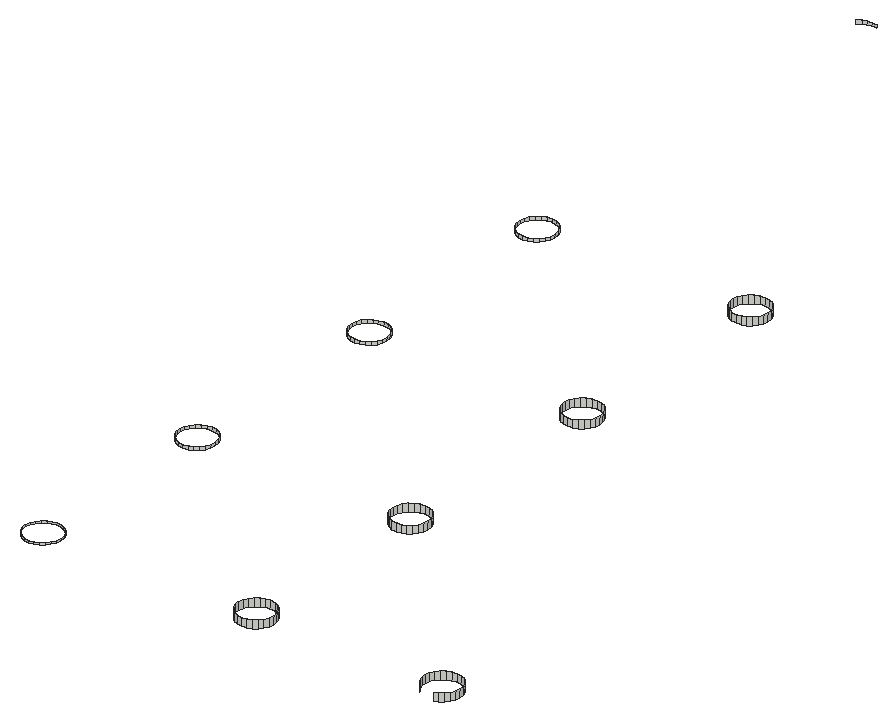
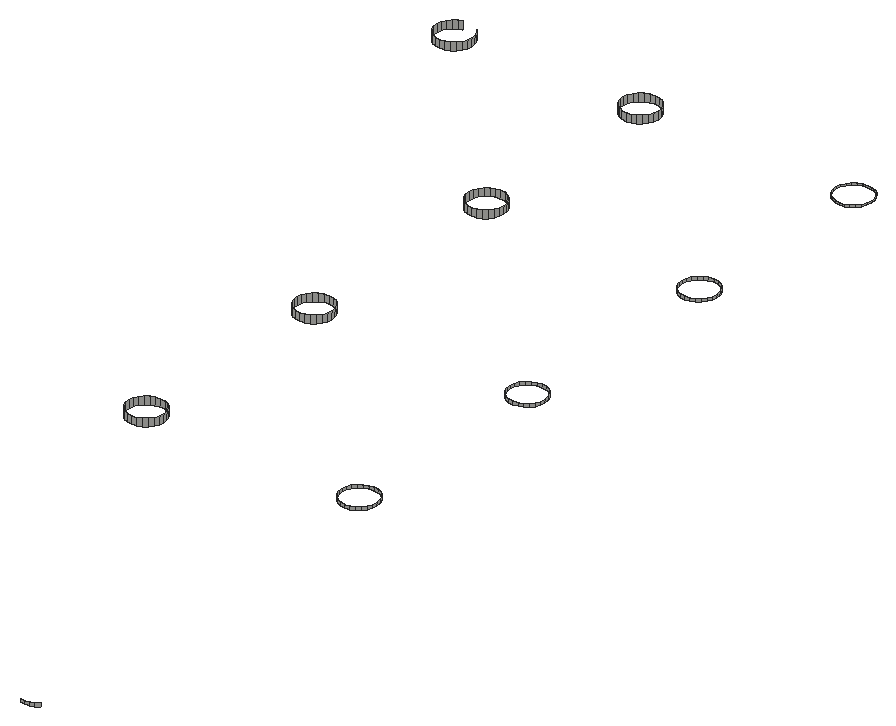
# SketchUp Ruby script. Lengths in inches.
U = 1.inch
M = Sketchup.active_model
def pt(a) = Geom::Point3d.new(a.map { |v| v * U })
def face(e, loops, mat)
  f = e.add_face(loops[0].map { |a| pt(a) })
  loops[1..].each { |l| e.add_face(l.map { |a| pt(a) }).erase! }
  f.material = f.back_material = mat if mat
  f
end
# faces: each face lists its corners as indices into pts; further lists are holes
def faces(e, pts, list, mat = nil) = list.each { |f| face(e, (f[0].is_a?(Array) ? f : [f]).map { |l| l.map { |i| pts[i] } }, mat) }
# xy, xz, yz: faces in a plane at the given z, y or x. An outline is a flat list of corners, or four numbers for a rectangle; further outlines are holes
def ring(l) = l.size == 4 ? [[l[0], l[1]], [l[2], l[1]], [l[2], l[3]], [l[0], l[3]]] : l.each_slice(2).to_a
def flat(e, list, mat, &to3) = list.each { |f| face(e, (f[0].is_a?(Array) ? f : [f]).map { |l| ring(l).map { |u, v| to3.(u, v) } }, mat) }
def xy(e, z, list, mat = nil) = flat(e, list, mat) { |x, y| [x, y, z] }
def xz(e, y, list, mat = nil) = flat(e, list, mat) { |x, z| [x, y, z] }
def yz(e, x, list, mat = nil) = flat(e, list, mat) { |y, z| [x, y, z] }
def lines(e, pts, list) = list.each { |a, b| e.add_line(pt(pts[a]), pt(pts[b])) }
# prism: a flat outline (further loops are holes) pulled along v
def prism(e, loops, v, mat = nil)
  f = face(e, loops, mat); d = Geom::Vector3d.new(v.map { |x| x * U })
  f.pushpull(f.normal.samedirection?(d) ? d.length : -d.length)
end
def box(e, o, s, mat = nil) = prism(e, [[o, [o[0] + s[0], o[1], o[2]], [o[0] + s[0], o[1] + s[1], o[2]], [o[0], o[1] + s[1], o[2]]]], [0, 0, s[2]], mat)
def at(x, y, z, deg = 0) = Geom::Transformation.translation(pt([x, y, z])) * Geom::Transformation.rotation(ORIGIN, Z_AXIS, deg.degrees)
def axes(o, x, y, z) = Geom::Transformation.new([*x, 0, *y, 0, *z, 0, *pt(o).to_a, 1])
def part(name) = M.definitions.add(name)
# library, detail: a bought-in or finely detailed component or shape, given as its bounding box
def library(name, o, s) = part(name).tap { |d| box(d.entities, o, s) }
def detail(e, o, s) = box(e.add_group.entities, o, s)
def put(e, d, t, mat = nil) = e.add_instance(d, t).tap { |i| i.material = mat if mat }
def group(e, t, mat = nil) = e.add_group.tap { |g| g.transformation = t; g.material = mat if mat }.entities
root = M.entities
p = [[271.15,385.12,126],[269.86,385.29,126],[269.86,385.29,126.5],[271.15,385.12,126.5],[272.44,385.29,126],[272.44,385.29,126.5],
  [331.21,385.12,126],[329.92,385.29,126],[329.92,385.29,128.125],[331.21,385.12,128.125],[332.51,385.29,126],[332.51,385.29,128.125],
  [268.65,385.79,126],[268.65,385.79,126.5],[273.65,385.79,126],[273.65,385.79,126.5],[328.71,385.79,126],[328.71,385.79,128.125],
  [333.71,385.79,126],[333.71,385.79,128.125],[386.27,385.79,126],[385.07,385.29,126],[385.07,385.29,128.125],[386.27,385.79,128.125],
  [267.61,386.58,126],[267.61,386.58,126.5],[274.68,386.58,126],[274.68,386.58,126.5],[327.68,386.58,126],[327.68,386.58,128.125],
  [334.75,386.58,126],[334.75,386.58,128.125],[387.31,386.58,126],[387.31,386.58,128.125],[266.82,387.62,126],[266.82,387.62,126.5],
  [275.48,387.62,126],[275.48,387.62,126.5],[326.88,387.62,126],[326.88,387.62,128.125],[335.54,387.62,126],[335.54,387.62,128.125],
  [380.24,386.58,126],[379.44,387.62,126],[379.44,387.62,128.125],[380.24,386.58,128.125],[388.1,387.62,126],[388.1,387.62,128.125],
  [266.32,388.83,126],[266.32,388.83,126.5],[275.98,388.83,126],[275.98,388.83,126.5],[326.38,388.83,126],[326.38,388.83,128.125],
  [336.04,388.83,126],[336.04,388.83,128.125],[378.94,388.83,126],[378.94,388.83,128.125],[388.6,388.83,126],[388.6,388.83,128.125],
  [266.15,390.12,126],[266.15,390.12,126.5],[276.15,390.12,126],[276.15,390.12,126.5],[326.21,390.12,126],[326.21,390.12,128.125],
  [336.21,390.12,126],[336.21,390.12,128.125],[378.77,390.12,126],[378.77,390.12,128.125],[388.77,390.12,126],[388.77,390.12,128.125],
  [266.32,391.41,126],[266.32,391.41,126.5],[275.98,391.41,126],[275.98,391.41,126.5],[326.38,391.41,126],[326.38,391.41,128.125],
  [336.04,391.41,126],[336.04,391.41,128.125],[378.94,391.41,126],[378.94,391.41,128.125],[388.6,391.41,126],[388.6,391.41,128.125],
  [266.82,392.62,126],[266.82,392.62,126.5],[275.48,392.62,126],[275.48,392.62,126.5],[326.88,392.62,126],[326.88,392.62,128.125],
  [335.54,392.62,126],[335.54,392.62,128.125],[379.44,392.62,126],[379.44,392.62,128.125],[388.1,392.62,126],[388.1,392.62,128.125],
  [267.61,393.66,126],[267.61,393.66,126.5],[274.68,393.66,126],[274.68,393.66,126.5],[327.68,393.66,126],[327.68,393.66,128.125],
  [334.75,393.66,126],[334.75,393.66,128.125],[380.24,393.66,126],[380.24,393.66,128.125],[387.31,393.66,126],[387.31,393.66,128.125],
  [268.65,394.45,126],[268.65,394.45,126.5],[273.65,394.45,126],[273.65,394.45,126.5],[328.71,394.45,126],[328.71,394.45,128.125],
  [333.71,394.45,126],[333.71,394.45,128.125],[381.27,394.45,126],[381.27,394.45,128.125],[386.27,394.45,126],[386.27,394.45,128.125],
  [269.86,394.95,126],[269.86,394.95,126.5],[272.44,394.95,126],[272.44,394.95,126.5],[329.92,394.95,126],[329.92,394.95,128.125],
  [332.51,394.95,126],[332.51,394.95,128.125],[382.48,394.95,126],[382.48,394.95,128.125],[385.07,394.95,126],[385.07,394.95,128.125],
  [271.15,395.12,126],[271.15,395.12,126.5],[331.21,395.12,126],[331.21,395.12,128.125],[383.77,395.12,126],[383.77,395.12,128.125],
  [271.15,439.5625,126],[269.86,439.73,126],[269.86,439.73,126.875],[271.15,439.5625,126.875],[272.44,439.73,126],[272.44,439.73,126.875],
  [331.21,439.5625,126],[329.92,439.73,126],[329.92,439.73,128.125],[331.21,439.5625,128.125],[332.51,439.73,126],[332.51,439.73,128.125],
  [268.65,440.23,126],[268.65,440.23,126.875],[273.65,440.23,126],[273.65,440.23,126.875],[328.71,440.23,126],[328.71,440.23,128.125],
  [333.71,440.23,126],[333.71,440.23,128.125],[267.61,441.03,126],[267.61,441.03,126.875],[274.68,441.03,126],[274.68,441.03,126.875],
  [327.68,441.03,126],[327.68,441.03,128.125],[334.75,441.03,126],[334.75,441.03,128.125],[266.82,442.0625,126],[266.82,442.0625,126.875],
  [275.48,442.0625,126],[275.48,442.0625,126.875],[326.88,442.0625,126],[326.88,442.0625,128.125],[335.54,442.0625,126],[335.54,442.0625,128.125],
  [266.32,443.27,126],[266.32,443.27,126.875],[275.98,443.27,126],[275.98,443.27,126.875],[326.38,443.27,126],[326.38,443.27,128.125],
  [336.04,443.27,126],[336.04,443.27,128.125],[266.15,444.5625,126],[266.15,444.5625,126.875],[276.15,444.5625,126],[276.15,444.5625,126.875],
  [326.21,444.5625,126],[326.21,444.5625,128.125],[336.21,444.5625,126],[336.21,444.5625,128.125],[266.32,445.86,126],[266.32,445.86,126.875],
  [275.98,445.86,126],[275.98,445.86,126.875],[326.38,445.86,126],[326.38,445.86,128.125],[336.04,445.86,126],[336.04,445.86,128.125],
  [266.82,447.0625,126],[266.82,447.0625,126.875],[275.48,447.0625,126],[275.48,447.0625,126.875],[326.88,447.0625,126],[326.88,447.0625,128.125],
  [335.54,447.0625,126],[335.54,447.0625,128.125],[267.61,448.1,126],[267.61,448.1,126.875],[274.68,448.1,126],[274.68,448.1,126.875],
  [327.68,448.1,126],[327.68,448.1,128.125],[334.75,448.1,126],[334.75,448.1,128.125],[268.65,448.89,126],[268.65,448.89,126.875],
  [273.65,448.89,126],[273.65,448.89,126.875],[328.71,448.89,126],[328.71,448.89,128.125],[333.71,448.89,126],[333.71,448.89,128.125],
  [269.86,449.39,126],[269.86,449.39,126.875],[272.44,449.39,126],[272.44,449.39,126.875],[329.92,449.39,126],[329.92,449.39,128.125],
  [332.51,449.39,126],[332.51,449.39,128.125],[271.15,449.5625,126],[271.15,449.5625,126.875],[331.21,449.5625,126],[331.21,449.5625,128.125],
  [271.15,500.05,126],[269.86,500.22,126],[269.86,500.22,126.875],[271.15,500.05,126.875],[272.44,500.22,126],[272.44,500.22,126.875],
  [331.21,500.05,126],[329.92,500.22,126],[329.92,500.22,128.125],[331.21,500.05,128.125],[332.51,500.22,126],[332.51,500.22,128.125],
  [268.65,500.72,126],[268.65,500.72,126.875],[273.65,500.72,126],[273.65,500.72,126.875],[328.71,500.72,126],[328.71,500.72,128.125],
  [333.71,500.72,126],[333.71,500.72,128.125],[267.61,501.52,126],[267.61,501.52,126.875],[274.68,501.52,126],[274.68,501.52,126.875],
  [327.68,501.52,126],[327.68,501.52,128.125],[334.75,501.52,126],[334.75,501.52,128.125],[266.82,502.55,126],[266.82,502.55,126.875],
  [275.48,502.55,126],[275.48,502.55,126.875],[326.88,502.55,126],[326.88,502.55,128.125],[335.54,502.55,126],[335.54,502.55,128.125],
  [266.32,503.76,126],[266.32,503.76,126.875],[275.98,503.76,126],[275.98,503.76,126.875],[326.38,503.76,126],[326.38,503.76,128.125],
  [336.04,503.76,126],[336.04,503.76,128.125],[266.15,505.05,126],[266.15,505.05,126.875],[276.15,505.05,126],[276.15,505.05,126.875],
  [326.21,505.05,126],[326.21,505.05,128.125],[336.21,505.05,126],[336.21,505.05,128.125],[266.32,506.35,126],[266.32,506.35,126.875],
  [275.98,506.35,126],[275.98,506.35,126.875],[326.38,506.35,126],[326.38,506.35,128.125],[336.04,506.35,126],[336.04,506.35,128.125],
  [266.82,507.55,126],[266.82,507.55,126.875],[275.48,507.55,126],[275.48,507.55,126.875],[326.88,507.55,126],[326.88,507.55,128.125],
  [335.54,507.55,126],[335.54,507.55,128.125],[267.61,508.59,126],[267.61,508.59,126.875],[274.68,508.59,126],[274.68,508.59,126.875],
  [327.68,508.59,126],[327.68,508.59,128.125],[334.75,508.59,126],[334.75,508.59,128.125],[268.65,509.38,126],[268.65,509.38,126.875],
  [273.65,509.38,126],[273.65,509.38,126.875],[328.71,509.38,126],[328.71,509.38,128.125],[333.71,509.38,126],[333.71,509.38,128.125],
  [269.86,509.88,126],[269.86,509.88,126.875],[272.44,509.88,126],[272.44,509.88,126.875],[329.92,509.88,126],[329.92,509.88,128.125],
  [332.51,509.88,126],[332.51,509.88,128.125],[271.15,510.05,126],[271.15,510.05,126.875],[331.21,510.05,126],[331.21,510.05,128.125],
  [271.15,559.33,126],[269.86,559.5,126],[269.86,559.5,126.875],[271.15,559.33,126.875],[272.44,559.5,126],[272.44,559.5,126.875],
  [331.21,559.33,126],[329.92,559.5,126],[329.92,559.5,128.125],[331.21,559.33,128.125],[332.51,559.5,126],[332.51,559.5,128.125],
  [268.65,560,126],[268.65,560,126.875],[273.65,560,126],[273.65,560,126.875],[328.71,560,126],[328.71,560,128.125],
  [333.71,560,126],[333.71,560,128.125],[267.61,560.79,126],[267.61,560.79,126.875],[274.68,560.79,126],[274.68,560.79,126.875],
  [327.68,560.79,126],[327.68,560.79,128.125],[334.75,560.79,126],[334.75,560.79,128.125],[266.82,561.83,126],[266.82,561.83,126.875],
  [275.48,561.83,126],[275.48,561.83,126.875],[326.88,561.83,126],[326.88,561.83,128.125],[335.54,561.83,126],[335.54,561.83,128.125],
  [266.32,563.03,126],[266.32,563.03,126.875],[275.98,563.03,126],[275.98,563.03,126.875],[326.38,563.03,126],[326.38,563.03,128.125],
  [336.04,563.03,126],[336.04,563.03,128.125],[266.15,564.33,126],[266.15,564.33,126.875],[276.15,564.33,126],[276.15,564.33,126.875],
  [326.21,564.33,126],[326.21,564.33,128.125],[336.21,564.33,126],[336.21,564.33,128.125],[266.32,565.62,126],[266.32,565.62,126.875],
  [275.98,565.62,126],[275.98,565.62,126.875],[326.38,565.62,126],[326.38,565.62,128.125],[336.04,565.62,126],[336.04,565.62,128.125],
  [266.82,566.83,126],[266.82,566.83,126.875],[275.48,566.83,126],[275.48,566.83,126.875],[326.88,566.83,126],[326.88,566.83,128.125],
  [335.54,566.83,126],[335.54,566.83,128.125],[267.61,567.86,126],[267.61,567.86,126.875],[274.68,567.86,126],[274.68,567.86,126.875],
  [327.68,567.86,126],[327.68,567.86,128.125],[334.75,567.86,126],[334.75,567.86,128.125],[268.65,568.66,126],[268.65,568.66,126.875],
  [273.65,568.66,126],[273.65,568.66,126.875],[328.71,568.66,126],[328.71,568.66,128.125],[333.71,568.66,126],[333.71,568.66,128.125],
  [269.86,569.16,126],[269.86,569.16,126.875],[272.44,569.16,126],[272.44,569.16,126.875],[329.92,569.16,126],[329.92,569.16,128.125],
  [332.51,569.16,126],[332.51,569.16,128.125],[271.15,569.33,126],[271.15,569.33,126.875],[331.21,569.33,126],[331.21,569.33,128.125],
  [267.61,680.8,126],[268.65,681.6,126],[268.65,681.6,126.875],[267.61,680.8,126.875],[269.86,682.1,126],[269.86,682.1,126.875],
  [271.15,682.27,126],[271.15,682.27,126.875],[272.44,682.1,126],[272.44,682.1,126.875]]
faces(root,p,[[0,1,2,3],[4,0,3,5],[6,7,8,9],[10,6,9,11],[1,12,13,2],[14,4,5,15],[7,16,17,8],[18,10,11,19],
  [20,21,22,23],[12,24,25,13],[26,14,15,27],[16,28,29,17],[30,18,19,31],[32,20,23,33],[24,34,35,25],[36,26,27,37],
  [28,38,39,29],[40,30,31,41],[42,43,44,45],[46,32,33,47],[34,48,49,35],[50,36,37,51],[38,52,53,39],[54,40,41,55],
  [43,56,57,44],[58,46,47,59],[48,60,61,49],[62,50,51,63],[52,64,65,53],[66,54,55,67],[56,68,69,57],[70,58,59,71],
  [60,72,73,61],[74,62,63,75],[64,76,77,65],[78,66,67,79],[68,80,81,69],[82,70,71,83],[72,84,85,73],[86,74,75,87],
  [76,88,89,77],[90,78,79,91],[80,92,93,81],[94,82,83,95],[84,96,97,85],[98,86,87,99],[88,100,101,89],[102,90,91,103],
  [92,104,105,93],[106,94,95,107],[96,108,109,97],[110,98,99,111],[100,112,113,101],[114,102,103,115],[104,116,117,105],[118,106,107,119],
  [108,120,121,109],[122,110,111,123],[112,124,125,113],[126,114,115,127],[116,128,129,117],[130,118,119,131],[120,132,133,121],[132,122,123,133],
  [124,134,135,125],[134,126,127,135],[128,136,137,129],[136,130,131,137],[138,139,140,141],[142,138,141,143],[144,145,146,147],[148,144,147,149],
  [139,150,151,140],[152,142,143,153],[145,154,155,146],[156,148,149,157],[150,158,159,151],[160,152,153,161],[154,162,163,155],[164,156,157,165],
  [158,166,167,159],[168,160,161,169],[162,170,171,163],[172,164,165,173],[166,174,175,167],[176,168,169,177],[170,178,179,171],[180,172,173,181],
  [174,182,183,175],[184,176,177,185],[178,186,187,179],[188,180,181,189],[182,190,191,183],[192,184,185,193],[186,194,195,187],[196,188,189,197],
  [190,198,199,191],[200,192,193,201],[194,202,203,195],[204,196,197,205],[198,206,207,199],[208,200,201,209],[202,210,211,203],[212,204,205,213],
  [206,214,215,207],[216,208,209,217],[210,218,219,211],[220,212,213,221],[214,222,223,215],[224,216,217,225],[218,226,227,219],[228,220,221,229],
  [222,230,231,223],[230,224,225,231],[226,232,233,227],[232,228,229,233],[234,235,236,237],[238,234,237,239],[240,241,242,243],[244,240,243,245],
  [235,246,247,236],[248,238,239,249],[241,250,251,242],[252,244,245,253],[246,254,255,247],[256,248,249,257],[250,258,259,251],[260,252,253,261],
  [254,262,263,255],[264,256,257,265],[258,266,267,259],[268,260,261,269],[262,270,271,263],[272,264,265,273],[266,274,275,267],[276,268,269,277],
  [270,278,279,271],[280,272,273,281],[274,282,283,275],[284,276,277,285],[278,286,287,279],[288,280,281,289],[282,290,291,283],[292,284,285,293],
  [286,294,295,287],[296,288,289,297],[290,298,299,291],[300,292,293,301],[294,302,303,295],[304,296,297,305],[298,306,307,299],[308,300,301,309],
  [302,310,311,303],[312,304,305,313],[306,314,315,307],[316,308,309,317],[310,318,319,311],[320,312,313,321],[314,322,323,315],[324,316,317,325],
  [318,326,327,319],[326,320,321,327],[322,328,329,323],[328,324,325,329],[330,331,332,333],[334,330,333,335],[336,337,338,339],[340,336,339,341],
  [331,342,343,332],[344,334,335,345],[337,346,347,338],[348,340,341,349],[342,350,351,343],[352,344,345,353],[346,354,355,347],[356,348,349,357],
  [350,358,359,351],[360,352,353,361],[354,362,363,355],[364,356,357,365],[358,366,367,359],[368,360,361,369],[362,370,371,363],[372,364,365,373],
  [366,374,375,367],[376,368,369,377],[370,378,379,371],[380,372,373,381],[374,382,383,375],[384,376,377,385],[378,386,387,379],[388,380,381,389],
  [382,390,391,383],[392,384,385,393],[386,394,395,387],[396,388,389,397],[390,398,399,391],[400,392,393,401],[394,402,403,395],[404,396,397,405],
  [398,406,407,399],[408,400,401,409],[402,410,411,403],[412,404,405,413],[406,414,415,407],[416,408,409,417],[410,418,419,411],[420,412,413,421],
  [414,422,423,415],[422,416,417,423],[418,424,425,419],[424,420,421,425],[426,427,428,429],[427,430,431,428],[430,432,433,431],[432,434,435,433]])
